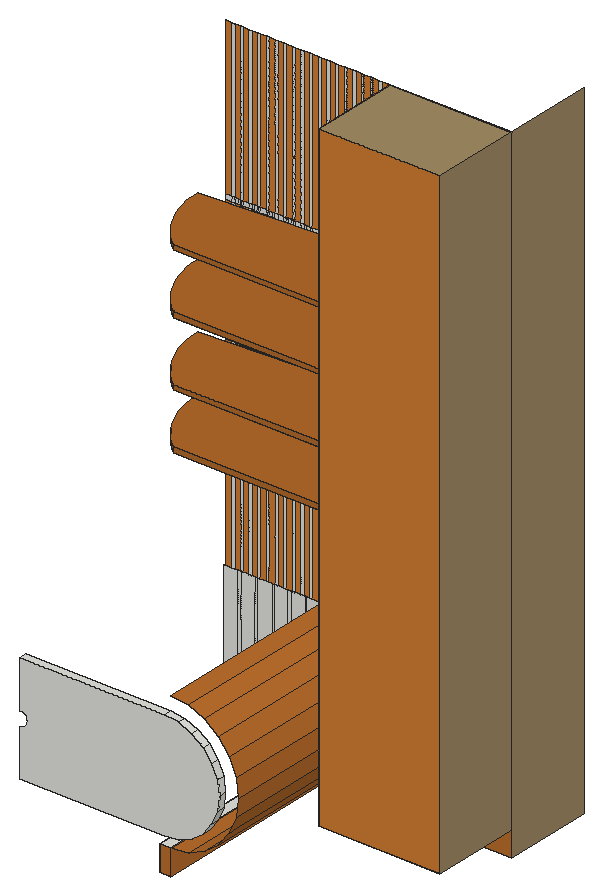
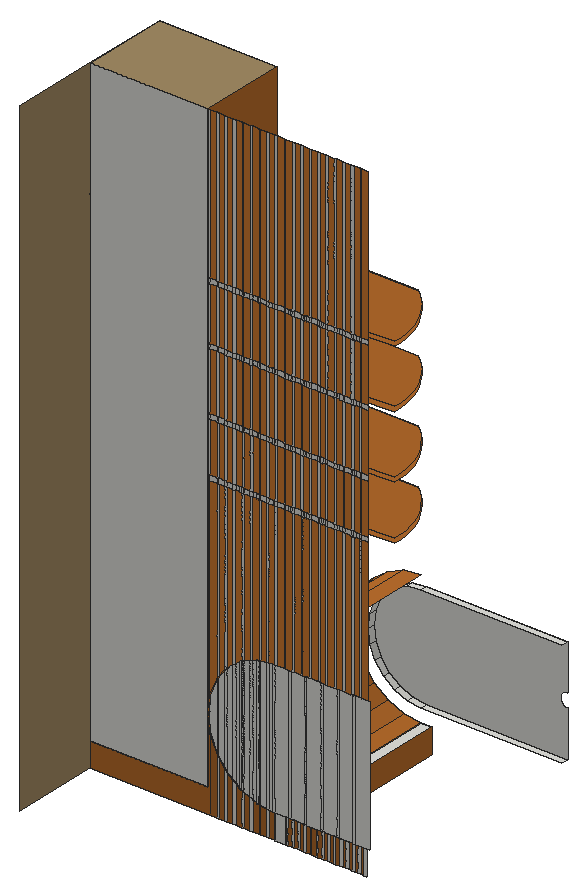
# SketchUp Ruby script. Lengths in inches.
U = 1.inch
M = Sketchup.active_model
def pt(a) = Geom::Point3d.new(a.map { |v| v * U })
def face(e, loops, mat)
  f = e.add_face(loops[0].map { |a| pt(a) })
  loops[1..].each { |l| e.add_face(l.map { |a| pt(a) }).erase! }
  f.material = f.back_material = mat if mat
  f
end
# faces: each face lists its corners as indices into pts; further lists are holes
def faces(e, pts, list, mat = nil) = list.each { |f| face(e, (f[0].is_a?(Array) ? f : [f]).map { |l| l.map { |i| pts[i] } }, mat) }
# xy, xz, yz: faces in a plane at the given z, y or x. An outline is a flat list of corners, or four numbers for a rectangle; further outlines are holes
def ring(l) = l.size == 4 ? [[l[0], l[1]], [l[2], l[1]], [l[2], l[3]], [l[0], l[3]]] : l.each_slice(2).to_a
def flat(e, list, mat, &to3) = list.each { |f| face(e, (f[0].is_a?(Array) ? f : [f]).map { |l| ring(l).map { |u, v| to3.(u, v) } }, mat) }
def xy(e, z, list, mat = nil) = flat(e, list, mat) { |x, y| [x, y, z] }
def xz(e, y, list, mat = nil) = flat(e, list, mat) { |x, z| [x, y, z] }
def yz(e, x, list, mat = nil) = flat(e, list, mat) { |y, z| [x, y, z] }
def lines(e, pts, list) = list.each { |a, b| e.add_line(pt(pts[a]), pt(pts[b])) }
# prism: a flat outline (further loops are holes) pulled along v
def prism(e, loops, v, mat = nil)
  f = face(e, loops, mat); d = Geom::Vector3d.new(v.map { |x| x * U })
  f.pushpull(f.normal.samedirection?(d) ? d.length : -d.length)
end
def box(e, o, s, mat = nil) = prism(e, [[o, [o[0] + s[0], o[1], o[2]], [o[0] + s[0], o[1] + s[1], o[2]], [o[0], o[1] + s[1], o[2]]]], [0, 0, s[2]], mat)
def at(x, y, z, deg = 0) = Geom::Transformation.translation(pt([x, y, z])) * Geom::Transformation.rotation(ORIGIN, Z_AXIS, deg.degrees)
def axes(o, x, y, z) = Geom::Transformation.new([*x, 0, *y, 0, *z, 0, *pt(o).to_a, 1])
def part(name) = M.definitions.add(name)
# library, detail: a bought-in or finely detailed component or shape, given as its bounding box
def library(name, o, s) = part(name).tap { |d| box(d.entities, o, s) }
def detail(e, o, s) = box(e.add_group.entities, o, s)
def put(e, d, t, mat = nil) = e.add_instance(d, t).tap { |i| i.material = mat if mat }
def group(e, t, mat = nil) = e.add_group.tap { |g| g.transformation = t; g.material = mat if mat }.entities
root = M.entities
M.materials.add("[Wood Bamboo]").color = [186, 110, 45]
M.materials.add("[Wood Bamboo]1").color = [211, 125, 51]
M.materials.add("[Wood Bamboo]2").color = [177, 105, 43]
M.materials.add("[Wood Floor Light]").color = [163, 140, 101]
xy(root,7.933,[[39.737,0.625,40.325,10.4375]],"[Wood Bamboo]")
xy(root,9.246,[[39.737,0.625,40.325,10.4375]])
xy(root,9.246,[[43.883,5.8125,50.1875,10.4375]],"[Wood Bamboo]")
xy(root,9.975,[[32.793,0.25,40.325,0.625]])
xy(root,15.633,[[32.793,0.25,40.325,0.625]])
xy(root,23.978,[[36.339,5.8125,36.045,6.057,35.77,6.324,35.516,6.611,35.285,6.916,35.077,7.238,34.895,7.575,34.739,7.925,34.61,8.285,34.509,8.655,34.437,9.031,34.393,9.411,34.378,9.794,34.378,10.4375,43.883,10.4375,43.883,5.8125]],"[Wood Bamboo]2")
xy(root,24.237,[[36.339,5.8125,43.883,5.8125,43.883,10.4375,34.378,10.4375,34.378,9.794,34.393,9.411,34.437,9.031,34.509,8.655,34.61,8.285,34.739,7.925,34.895,7.575,35.077,7.238,35.285,6.916,35.516,6.611,35.77,6.324,36.045,6.057]],"[Wood Bamboo]2")
xy(root,26.915,[[36.339,5.8125,36.045,6.057,35.77,6.324,35.516,6.611,35.285,6.916,35.077,7.238,34.895,7.575,34.739,7.925,34.61,8.285,34.509,8.655,34.437,9.031,34.393,9.411,34.378,9.794,34.378,10.4375,43.883,10.4375,43.883,5.8125]],"[Wood Bamboo]2")
xy(root,27.175,[[36.339,5.8125,43.883,5.8125,43.883,10.4375,34.378,10.4375,34.378,9.794,34.393,9.411,34.437,9.031,34.509,8.655,34.61,8.285,34.739,7.925,34.895,7.575,35.077,7.238,35.285,6.916,35.516,6.611,35.77,6.324,36.045,6.057]],"[Wood Bamboo]2")
xy(root,30.29,[[36.339,5.8125,36.045,6.057,35.77,6.324,35.516,6.611,35.285,6.916,35.077,7.238,34.895,7.575,34.739,7.925,34.61,8.285,34.509,8.655,34.437,9.031,34.393,9.411,34.378,9.794,34.378,10.4375,43.883,10.4375,43.883,5.8125]],"[Wood Bamboo]2")
xy(root,30.55,[[36.339,5.8125,43.883,5.8125,43.883,10.4375,34.378,10.4375,34.378,9.794,34.393,9.411,34.437,9.031,34.509,8.655,34.61,8.285,34.739,7.925,34.895,7.575,35.077,7.238,35.285,6.916,35.516,6.611,35.77,6.324,36.045,6.057]],"[Wood Bamboo]2")
xy(root,33.415,[[36.339,5.8125,36.045,6.057,35.77,6.324,35.516,6.611,35.285,6.916,35.077,7.238,34.895,7.575,34.739,7.925,34.61,8.285,34.509,8.655,34.437,9.031,34.393,9.411,34.378,9.794,34.378,10.4375,43.883,10.4375,43.883,5.8125]],"[Wood Bamboo]2")
xy(root,33.675,[[36.339,5.8125,43.883,5.8125,43.883,10.4375,34.378,10.4375,34.378,9.794,34.393,9.411,34.437,9.031,34.509,8.655,34.61,8.285,34.739,7.925,34.895,7.575,35.077,7.238,35.285,6.916,35.516,6.611,35.77,6.324,36.045,6.057]],"[Wood Bamboo]2")
xy(root,41.746,[[43.883,5.8125,50.1875,10.4375]],"[Wood Floor Light]")
xz(root,0.25,[[32.793,9.975,40.325,9.975,41.057,10.071,41.74,10.354,42.326,10.803,42.775,11.389,43.058,12.072,43.154,12.804,43.058,13.536,42.775,14.219,42.326,14.805,41.74,15.254,41.057,15.537,40.325,15.633,32.793,15.633,32.793,13.179,32.89,13.166,32.98,13.129,33.058,13.069,33.117,12.992,33.155,12.901,33.168,12.804,33.155,12.707,33.117,12.617,33.058,12.539,32.98,12.479,32.89,12.442,32.793,12.429]])
xz(root,0.625,[[39.737,7.933,40.325,9.246]],"[Wood Bamboo]")
xz(root,5.8125,[[43.883,9.246,50.1875,41.746]],"[Wood Bamboo]1")
xz(root,5.8125,[[36.339,23.978,43.883,24.237],[36.339,26.915,43.883,27.175],[36.339,30.29,43.883,30.55],[36.339,33.415,43.883,33.675]],"[Wood Bamboo]2")
xz(root,10.4375,[[35.398,7.933,35.523,9.246],[35.722,7.933,35.847,9.246],[36.046,7.933,36.171,9.246],[36.37,7.933,36.495,9.246],[36.695,7.933,36.82,9.246],
  [37.019,7.933,37.144,9.246],[37.343,7.933,37.468,9.246],[37.667,7.933,37.792,9.246],[37.991,7.933,38.116,9.246],[38.315,7.933,38.44,9.246],
  [38.639,7.933,38.764,9.246],[38.964,7.933,39.089,9.246],[39.288,7.933,39.413,9.246],[39.612,7.933,39.737,9.246],[39.737,7.933,40.303,9.246],
  [40.303,7.933,40.325,9.246],[40.605,7.933,40.73,7.933,40.73,9.299,40.605,9.283],[41.056,7.933,41.181,7.933,41.181,9.358,41.166,9.357,41.056,9.342],[41.506,7.933,41.631,7.933,41.631,9.527,41.506,9.475],[41.957,7.933,42.082,7.933,42.082,9.713,42.03,9.692,41.957,9.661],
  [42.407,7.933,42.532,7.933,42.532,10.051,42.407,9.955],[42.857,7.933,42.982,7.933,42.982,10.472,42.894,10.357,42.857,10.309],[43.308,7.933,43.433,7.933,43.433,11.088,43.407,11.025,43.308,10.896],[35.244,9.246,35.983,16.362],[35.983,9.246,36.108,16.362],
  [36.108,9.246,36.847,16.362],[36.847,9.246,36.972,16.362],[36.972,9.246,37.711,16.362],[37.711,9.246,37.836,16.362],[37.836,9.246,38.575,16.362],
  [38.575,9.246,38.7,16.362],[38.7,9.246,39.439,16.362],[39.439,9.246,39.564,16.362],[39.564,9.246,40.303,16.362],[40.303,9.246,40.325,9.246,40.428,9.259,40.428,16.349,40.325,16.362,40.303,16.362],
  [43.883,9.246,50.1875,41.746],[40.428,9.259,40.428,16.349,40.605,16.325,40.605,9.283],[40.605,9.283,40.605,16.325,40.73,16.309,40.73,9.299],[40.73,9.299,40.73,16.309,41.056,16.266,41.056,9.342],[41.056,9.342,41.056,16.266,41.166,16.251,41.166,9.357],
  [41.166,9.357,41.181,9.358,41.181,16.25,41.166,16.251],[41.181,9.358,41.246,9.367,41.291,9.386,41.291,16.222,41.246,16.241,41.181,16.25],[41.291,9.386,41.291,16.222,41.506,16.133,41.506,9.475],[41.506,9.475,41.506,16.133,41.631,16.081,41.631,9.527],[41.631,9.527,41.631,16.081,41.957,15.947,41.957,9.661],
  [41.957,9.661,41.957,15.947,42.03,15.916,42.03,9.692],[42.03,9.692,42.082,9.713,42.082,15.895,42.03,15.916],[42.082,9.713,42.104,9.723,42.155,9.762,42.155,15.846,42.104,15.886,42.082,15.895],[42.155,9.762,42.155,15.846,42.407,15.653,42.407,9.955],[42.407,9.955,42.407,15.653,42.532,15.557,42.532,10.051],
  [42.532,10.051,42.532,15.557,42.841,15.32,42.857,15.299,42.857,10.309,42.841,10.288],[42.857,10.309,42.857,15.299,42.894,15.251,42.894,10.357],[42.894,10.357,42.982,10.472,42.982,15.136,42.894,15.251],[42.982,10.472,43.019,10.52,43.019,15.088,42.982,15.136],[43.019,10.52,43.019,15.088,43.308,14.712,43.308,10.896],
  [43.308,10.896,43.308,14.712,43.407,14.583,43.433,14.52,43.433,11.088,43.407,11.025],[43.433,11.088,43.433,14.52,43.758,13.734,43.758,11.874],[43.758,11.874,43.758,13.734,43.762,13.725,43.883,12.804,43.762,11.883],[43.758,11.874,43.762,11.883,43.883,12.804,43.762,13.725,43.758,13.734],[43.883,12.804,43.883,23.978,43.758,23.978,43.758,13.734,43.762,13.725],
  [43.433,14.52,43.433,23.978,43.308,23.978,43.308,14.712,43.407,14.583],[42.982,15.136,42.982,23.978,42.857,23.978,42.857,15.299,42.894,15.251],[42.532,15.557,42.532,23.978,42.407,23.978,42.407,15.653],[42.082,15.895,42.082,23.978,41.957,23.978,41.957,15.947,42.03,15.916],[41.631,16.081,41.631,23.978,41.506,23.978,41.506,16.133],
  [41.181,16.25,41.181,23.978,41.056,23.978,41.056,16.266,41.166,16.251],[40.73,16.309,40.73,23.978,40.605,23.978,40.605,16.325],[35.65,16.362,35.775,23.978],[36.101,16.362,36.226,23.978],[36.551,16.362,36.676,23.978],
  [37.002,16.362,37.127,23.978],[37.452,16.362,37.577,23.978],[37.903,16.362,38.028,23.978],[38.353,16.362,38.478,23.978],[38.804,16.362,38.929,23.978],
  [39.254,16.362,39.379,23.978],[39.704,16.362,39.829,23.978],[40.155,16.362,40.28,23.978],[35.325,23.978,35.65,24.237],[35.65,23.978,35.775,24.237],
  [35.775,23.978,35.983,24.237],[35.983,23.978,36.101,24.237],[36.101,23.978,36.108,24.237],[36.108,23.978,36.226,24.237],[36.226,23.978,36.551,24.237],
  [36.551,23.978,36.676,24.237],[36.676,23.978,36.847,24.237],[36.847,23.978,36.972,24.237],[36.972,23.978,37.002,24.237],[37.002,23.978,37.127,24.237],
  [37.127,23.978,37.452,24.237],[37.452,23.978,37.577,24.237],[37.577,23.978,37.711,24.237],[37.711,23.978,37.836,24.237],[37.836,23.978,37.903,24.237],
  [37.903,23.978,38.028,24.237],[38.028,23.978,38.353,24.237],[38.353,23.978,38.478,24.237],[38.478,23.978,38.575,24.237],[38.575,23.978,38.7,24.237],
  [38.7,23.978,38.804,24.237],[38.804,23.978,38.929,24.237],[38.929,23.978,39.254,24.237],[39.254,23.978,39.379,24.237],[39.379,23.978,39.439,24.237],
  [39.439,23.978,39.564,24.237],[39.564,23.978,39.704,24.237],[39.704,23.978,39.829,24.237],[39.829,23.978,40.155,24.237],[40.155,23.978,40.28,24.237],
  [40.28,23.978,40.303,24.237],[40.303,23.978,40.428,24.237],[40.428,23.978,40.605,24.237],[40.605,23.978,40.73,24.237],[40.73,23.978,41.056,24.237],
  [41.056,23.978,41.166,24.237],[41.166,23.978,41.181,24.237],[41.181,23.978,41.291,24.237],[41.291,23.978,41.506,24.237],[41.506,23.978,41.631,24.237],
  [41.631,23.978,41.957,24.237],[41.957,23.978,42.03,24.237],[42.03,23.978,42.082,24.237],[42.082,23.978,42.155,24.237],[42.155,23.978,42.407,24.237],
  [42.407,23.978,42.532,24.237],[42.532,23.978,42.857,24.237],[42.857,23.978,42.894,24.237],[42.894,23.978,42.982,24.237],[42.982,23.978,43.019,24.237],
  [43.019,23.978,43.308,24.237],[43.308,23.978,43.433,24.237],[43.433,23.978,43.758,24.237],[43.758,23.978,43.883,24.237],[35.65,24.237,35.775,26.915],
  [36.101,24.237,36.226,26.915],[36.551,24.237,36.676,26.915],[37.002,24.237,37.127,26.915],[37.452,24.237,37.577,26.915],[37.903,24.237,38.028,26.915],
  [38.353,24.237,38.478,26.915],[38.804,24.237,38.929,26.915],[39.254,24.237,39.379,26.915],[39.704,24.237,39.829,26.915],[40.155,24.237,40.28,26.915],
  [40.605,24.237,40.73,26.915],[41.056,24.237,41.181,26.915],[41.506,24.237,41.631,26.915],[41.957,24.237,42.082,26.915],[42.407,24.237,42.532,26.915],
  [42.857,24.237,42.982,26.915],[43.308,24.237,43.433,26.915],[43.758,24.237,43.883,26.915],[35.325,26.915,35.65,27.175],[35.65,26.915,35.775,27.175],
  [35.775,26.915,35.983,27.175],[35.983,26.915,36.101,27.175],[36.101,26.915,36.108,27.175],[36.108,26.915,36.226,27.175],[36.226,26.915,36.551,27.175],
  [36.551,26.915,36.676,27.175],[36.676,26.915,36.847,27.175],[36.847,26.915,36.972,27.175],[36.972,26.915,37.002,27.175],[37.002,26.915,37.127,27.175],
  [37.127,26.915,37.452,27.175],[37.452,26.915,37.577,27.175],[37.577,26.915,37.711,27.175],[37.711,26.915,37.836,27.175],[37.836,26.915,37.903,27.175],
  [37.903,26.915,38.028,27.175],[38.028,26.915,38.353,27.175],[38.353,26.915,38.478,27.175],[38.478,26.915,38.575,27.175],[38.575,26.915,38.7,27.175],
  [38.7,26.915,38.804,27.175],[38.804,26.915,38.929,27.175],[38.929,26.915,39.254,27.175],[39.254,26.915,39.379,27.175],[39.379,26.915,39.439,27.175],
  [39.439,26.915,39.564,27.175],[39.564,26.915,39.704,27.175],[39.704,26.915,39.829,27.175],[39.829,26.915,40.155,27.175],[40.155,26.915,40.28,27.175],
  [40.28,26.915,40.303,27.175],[40.303,26.915,40.428,27.175],[40.428,26.915,40.605,27.175],[40.605,26.915,40.73,27.175],[40.73,26.915,41.056,27.175],
  [41.056,26.915,41.166,27.175],[41.166,26.915,41.181,27.175],[41.181,26.915,41.291,27.175],[41.291,26.915,41.506,27.175],[41.506,26.915,41.631,27.175],
  [41.631,26.915,41.957,27.175],[41.957,26.915,42.03,27.175],[42.03,26.915,42.082,27.175],[42.082,26.915,42.155,27.175],[42.155,26.915,42.407,27.175],
  [42.407,26.915,42.532,27.175],[42.532,26.915,42.857,27.175],[42.857,26.915,42.894,27.175],[42.894,26.915,42.982,27.175],[42.982,26.915,43.019,27.175],
  [43.019,26.915,43.308,27.175],[43.308,26.915,43.433,27.175],[43.433,26.915,43.758,27.175],[43.758,26.915,43.883,27.175],[35.65,27.175,35.775,30.29],
  [36.101,27.175,36.226,30.29],[36.551,27.175,36.676,30.29],[37.002,27.175,37.127,30.29],[37.452,27.175,37.577,30.29],[37.903,27.175,38.028,30.29],
  [38.353,27.175,38.478,30.29],[38.804,27.175,38.929,30.29],[39.254,27.175,39.379,30.29],[39.704,27.175,39.829,30.29],[40.155,27.175,40.28,30.29],
  [40.605,27.175,40.73,30.29],[41.056,27.175,41.181,30.29],[41.506,27.175,41.631,30.29],[41.957,27.175,42.082,30.29],[42.407,27.175,42.532,30.29],
  [42.857,27.175,42.982,30.29],[43.308,27.175,43.433,30.29],[43.758,27.175,43.883,30.29],[35.325,30.29,35.65,30.55],[35.65,30.29,35.775,30.55],
  [35.775,30.29,35.983,30.55],[35.983,30.29,36.101,30.55],[36.101,30.29,36.108,30.55],[36.108,30.29,36.226,30.55],[36.226,30.29,36.551,30.55],
  [36.551,30.29,36.676,30.55],[36.676,30.29,36.847,30.55],[36.847,30.29,36.972,30.55],[36.972,30.29,37.002,30.55],[37.002,30.29,37.127,30.55],
  [37.127,30.29,37.452,30.55],[37.452,30.29,37.577,30.55],[37.577,30.29,37.711,30.55],[37.711,30.29,37.836,30.55],[37.836,30.29,37.903,30.55],
  [37.903,30.29,38.028,30.55],[38.028,30.29,38.353,30.55],[38.353,30.29,38.478,30.55],[38.478,30.29,38.575,30.55],[38.575,30.29,38.7,30.55],
  [38.7,30.29,38.804,30.55],[38.804,30.29,38.929,30.55],[38.929,30.29,39.254,30.55],[39.254,30.29,39.379,30.55],[39.379,30.29,39.439,30.55],
  [39.439,30.29,39.564,30.55],[39.564,30.29,39.704,30.55],[39.704,30.29,39.829,30.55],[39.829,30.29,40.155,30.55],[40.155,30.29,40.28,30.55],
  [40.28,30.29,40.303,30.55],[40.303,30.29,40.428,30.55],[40.428,30.29,40.605,30.55],[40.605,30.29,40.73,30.55],[40.73,30.29,41.056,30.55],
  [41.056,30.29,41.166,30.55],[41.166,30.29,41.181,30.55],[41.181,30.29,41.291,30.55],[41.291,30.29,41.506,30.55],[41.506,30.29,41.631,30.55],
  [41.631,30.29,41.957,30.55],[41.957,30.29,42.03,30.55],[42.03,30.29,42.082,30.55],[42.082,30.29,42.155,30.55],[42.155,30.29,42.407,30.55],
  [42.407,30.29,42.532,30.55],[42.532,30.29,42.857,30.55],[42.857,30.29,42.894,30.55],[42.894,30.29,42.982,30.55],[42.982,30.29,43.019,30.55],
  [43.019,30.29,43.308,30.55],[43.308,30.29,43.433,30.55],[43.433,30.29,43.758,30.55],[43.758,30.29,43.883,30.55],[35.65,30.55,35.775,33.415],
  [36.101,30.55,36.226,33.415],[36.551,30.55,36.676,33.415],[37.002,30.55,37.127,33.415],[37.452,30.55,37.577,33.415],[37.903,30.55,38.028,33.415],
  [38.353,30.55,38.478,33.415],[38.804,30.55,38.929,33.415],[39.254,30.55,39.379,33.415],[39.704,30.55,39.829,33.415],[40.155,30.55,40.28,33.415],
  [40.605,30.55,40.73,33.415],[41.056,30.55,41.181,33.415],[41.506,30.55,41.631,33.415],[41.957,30.55,42.082,33.415],[42.407,30.55,42.532,33.415],
  [42.857,30.55,42.982,33.415],[43.308,30.55,43.433,33.415],[43.758,30.55,43.883,33.415],[35.325,33.415,35.65,33.675],[35.65,33.415,35.775,33.675],
  [35.775,33.415,35.983,33.675],[35.983,33.415,36.101,33.675],[36.101,33.415,36.108,33.675],[36.108,33.415,36.226,33.675],[36.226,33.415,36.551,33.675],
  [36.551,33.415,36.676,33.675],[36.676,33.415,36.847,33.675],[36.847,33.415,36.972,33.675],[36.972,33.415,37.002,33.675],[37.002,33.415,37.127,33.675],
  [37.127,33.415,37.452,33.675],[37.452,33.415,37.577,33.675],[37.577,33.415,37.711,33.675],[37.711,33.415,37.836,33.675],[37.836,33.415,37.903,33.675],
  [37.903,33.415,38.028,33.675],[38.028,33.415,38.353,33.675],[38.353,33.415,38.478,33.675],[38.478,33.415,38.575,33.675],[38.575,33.415,38.7,33.675],
  [38.7,33.415,38.804,33.675],[38.804,33.415,38.929,33.675],[38.929,33.415,39.254,33.675],[39.254,33.415,39.379,33.675],[39.379,33.415,39.439,33.675],
  [39.439,33.415,39.564,33.675],[39.564,33.415,39.704,33.675],[39.704,33.415,39.829,33.675],[39.829,33.415,40.155,33.675],[40.155,33.415,40.28,33.675],
  [40.28,33.415,40.303,33.675],[40.303,33.415,40.428,33.675],[40.428,33.415,40.605,33.675],[40.605,33.415,40.73,33.675],[40.73,33.415,41.056,33.675],
  [41.056,33.415,41.166,33.675],[41.166,33.415,41.181,33.675],[41.181,33.415,41.291,33.675],[41.291,33.415,41.506,33.675],[41.506,33.415,41.631,33.675],
  [41.631,33.415,41.957,33.675],[41.957,33.415,42.03,33.675],[42.03,33.415,42.082,33.675],[42.082,33.415,42.155,33.675],[42.155,33.415,42.407,33.675],
  [42.407,33.415,42.532,33.675],[42.532,33.415,42.857,33.675],[42.857,33.415,42.894,33.675],[42.894,33.415,42.982,33.675],[42.982,33.415,43.019,33.675],
  [43.019,33.415,43.308,33.675],[43.308,33.415,43.433,33.675],[43.433,33.415,43.758,33.675],[43.758,33.415,43.883,33.675],[35.65,33.675,35.775,41.746],
  [36.101,33.675,36.226,41.746],[36.551,33.675,36.676,41.746],[37.002,33.675,37.127,41.746],[37.452,33.675,37.577,41.746],[37.903,33.675,38.028,41.746],
  [38.353,33.675,38.478,41.746],[38.804,33.675,38.929,41.746],[39.254,33.675,39.379,41.746],[39.704,33.675,39.829,41.746],[40.155,33.675,40.28,41.746],
  [40.605,33.675,40.73,41.746],[41.056,33.675,41.181,41.746],[41.506,33.675,41.631,41.746],[41.957,33.675,42.082,41.746],[42.407,33.675,42.532,41.746],
  [42.857,33.675,42.982,41.746],[43.308,33.675,43.433,41.746],[43.758,33.675,43.883,41.746]])
xz(root,10.4375,[[43.758,7.933,50.1875,7.933,50.1875,9.246,43.883,9.246,43.883,12.804,43.762,11.883,43.758,11.874]],"[Wood Bamboo]")
xz(root,10.4375,[[43.758,13.734,43.758,23.978,43.433,23.978,43.433,14.52],[43.308,14.712,43.308,23.978,42.982,23.978,42.982,15.136,43.019,15.088],[42.857,15.299,42.857,23.978,42.532,23.978,42.532,15.557,42.841,15.32],[42.407,15.653,42.407,23.978,42.082,23.978,42.082,15.895,42.104,15.886,42.155,15.846],[41.957,15.947,41.957,23.978,41.631,23.978,41.631,16.081],
  [41.506,16.133,41.506,23.978,41.181,23.978,41.181,16.25,41.246,16.241,41.291,16.222],[41.056,16.266,41.056,23.978,40.73,23.978,40.73,16.309],[40.605,16.325,40.605,23.978,40.28,23.978,40.28,16.362,40.325,16.362,40.428,16.349],[35.325,16.362,35.65,23.978],[35.775,16.362,36.101,23.978],
  [36.226,16.362,36.551,23.978],[36.676,16.362,37.002,23.978],[37.127,16.362,37.452,23.978],[37.577,16.362,37.903,23.978],[38.028,16.362,38.353,23.978],
  [38.478,16.362,38.804,23.978],[38.929,16.362,39.254,23.978],[39.379,16.362,39.704,23.978],[39.829,16.362,40.155,23.978],[35.325,24.237,35.65,26.915],
  [35.775,24.237,36.101,26.915],[36.226,24.237,36.551,26.915],[36.676,24.237,37.002,26.915],[37.127,24.237,37.452,26.915],[37.577,24.237,37.903,26.915],
  [38.028,24.237,38.353,26.915],[38.478,24.237,38.804,26.915],[38.929,24.237,39.254,26.915],[39.379,24.237,39.704,26.915],[39.829,24.237,40.155,26.915],
  [40.28,24.237,40.605,26.915],[40.73,24.237,41.056,26.915],[41.181,24.237,41.506,26.915],[41.631,24.237,41.957,26.915],[42.082,24.237,42.407,26.915],
  [42.532,24.237,42.857,26.915],[42.982,24.237,43.308,26.915],[43.433,24.237,43.758,26.915],[35.325,27.175,35.65,30.29],[35.775,27.175,36.101,30.29],
  [36.226,27.175,36.551,30.29],[36.676,27.175,37.002,30.29],[37.127,27.175,37.452,30.29],[37.577,27.175,37.903,30.29],[38.028,27.175,38.353,30.29],
  [38.478,27.175,38.804,30.29],[38.929,27.175,39.254,30.29],[39.379,27.175,39.704,30.29],[39.829,27.175,40.155,30.29],[40.28,27.175,40.605,30.29],
  [40.73,27.175,41.056,30.29],[41.181,27.175,41.506,30.29],[41.631,27.175,41.957,30.29],[42.082,27.175,42.407,30.29],[42.532,27.175,42.857,30.29],
  [42.982,27.175,43.308,30.29],[43.433,27.175,43.758,30.29],[35.325,30.55,35.65,33.415],[35.775,30.55,36.101,33.415],[36.226,30.55,36.551,33.415],
  [36.676,30.55,37.002,33.415],[37.127,30.55,37.452,33.415],[37.577,30.55,37.903,33.415],[38.028,30.55,38.353,33.415],[38.478,30.55,38.804,33.415],
  [38.929,30.55,39.254,33.415],[39.379,30.55,39.704,33.415],[39.829,30.55,40.155,33.415],[40.28,30.55,40.605,33.415],[40.73,30.55,41.056,33.415],
  [41.181,30.55,41.506,33.415],[41.631,30.55,41.957,33.415],[42.082,30.55,42.407,33.415],[42.532,30.55,42.857,33.415],[42.982,30.55,43.308,33.415],
  [43.433,30.55,43.758,33.415],[35.325,33.675,35.65,41.746],[35.775,33.675,36.101,41.746],[36.226,33.675,36.551,41.746],[36.676,33.675,37.002,41.746],
  [37.127,33.675,37.452,41.746],[37.577,33.675,37.903,41.746],[38.028,33.675,38.353,41.746],[38.478,33.675,38.804,41.746],[38.929,33.675,39.254,41.746],
  [39.379,33.675,39.704,41.746],[39.829,33.675,40.155,41.746],[40.28,33.675,40.605,41.746],[40.73,33.675,41.056,41.746],[41.181,33.675,41.506,41.746],
  [41.631,33.675,41.957,41.746],[42.082,33.675,42.407,41.746],[42.532,33.675,42.857,41.746],[42.982,33.675,43.308,41.746],[43.433,33.675,43.758,41.746]],"[Wood Bamboo]1")
xz(root,10.4375,[[35.523,7.933,35.722,9.246],[35.847,7.933,36.046,9.246],[36.171,7.933,36.37,9.246],[36.495,7.933,36.695,9.246],[36.82,7.933,37.019,9.246],
  [37.144,7.933,37.343,9.246],[37.468,7.933,37.667,9.246],[37.792,7.933,37.991,9.246],[38.116,7.933,38.315,9.246],[38.44,7.933,38.639,9.246],
  [38.764,7.933,38.964,9.246],[39.089,7.933,39.288,9.246],[39.413,7.933,39.612,9.246],[40.325,7.933,40.605,7.933,40.605,9.283,40.428,9.259,40.325,9.246],[40.73,7.933,41.056,7.933,41.056,9.342,40.73,9.299],
  [41.181,7.933,41.506,7.933,41.506,9.475,41.291,9.386,41.246,9.367,41.181,9.358],[41.631,7.933,41.957,7.933,41.957,9.661,41.631,9.527],[42.082,7.933,42.407,7.933,42.407,9.955,42.155,9.762,42.104,9.723,42.082,9.713],[42.532,7.933,42.857,7.933,42.857,10.309,42.841,10.288,42.532,10.051],[42.982,7.933,43.308,7.933,43.308,10.896,43.019,10.52,42.982,10.472],
  [43.433,7.933,43.758,7.933,43.758,11.874,43.433,11.088]],"[Wood Bamboo]2")
yz(root,39.737,[[0.625,7.933,10.4375,9.246]],"[Wood Bamboo]")
yz(root,40.325,[[0.625,7.933,10.4375,9.246]],"[Wood Bamboo]")
yz(root,43.883,[[5.8125,23.978,10.4375,24.237],[5.8125,26.915,10.4375,27.175],[5.8125,30.29,10.4375,30.55],[5.8125,33.415,10.4375,33.675]])
yz(root,43.883,[[5.8125,33.675,10.4375,41.746]],"[Wood Bamboo]")
yz(root,43.883,[[5.8125,12.804,10.4375,23.978],[5.8125,24.237,10.4375,26.915],[5.8125,27.175,10.4375,30.29],[5.8125,30.55,10.4375,33.415]],"[Wood Bamboo]1")
yz(root,43.883,[[5.8125,9.246,10.4375,12.804]],"[Wood Bamboo]2")
yz(root,50.1875,[[10.4375,7.933,15.125,41.746],[5.8125,9.246,10.4375,41.746]],"[Wood Floor Light]")
p = [[40.325,10.4375,9.246],[40.428,10.4375,9.259],[40.605,10.4375,9.283],[40.73,10.4375,9.299],[41.056,10.4375,9.342],[41.166,10.4375,9.357],
  [41.181,10.4375,9.358],[41.246,10.4375,9.367],[41.246,0.625,9.367],[40.325,0.625,9.246],[41.291,10.4375,9.386],[41.506,10.4375,9.475],
  [41.631,10.4375,9.527],[41.957,10.4375,9.661],[42.03,10.4375,9.692],[42.082,10.4375,9.713],[42.104,10.4375,9.723],[42.104,0.625,9.723],
  [42.155,10.4375,9.762],[42.407,10.4375,9.955],[42.532,10.4375,10.051],[42.841,10.4375,10.288],[42.841,0.625,10.288],[40.325,0.625,9.975],
  [41.057,0.625,10.071],[41.057,0.25,10.071],[40.325,0.25,9.975],[41.74,0.625,10.354],[41.74,0.25,10.354],[42.857,10.4375,10.309],
  [42.894,10.4375,10.357],[42.982,10.4375,10.472],[43.019,10.4375,10.52],[43.308,10.4375,10.896],[43.407,10.4375,11.025],[43.407,0.625,11.025],
  [42.326,0.625,10.803],[42.326,0.25,10.803],[42.775,0.625,11.389],[42.775,0.25,11.389],[43.433,10.4375,11.088],[43.758,10.4375,11.874],
  [43.762,10.4375,11.883],[43.762,0.625,11.883],[43.058,0.625,12.072],[43.058,0.25,12.072],[43.883,10.4375,12.804],[43.883,5.8125,12.804],
  [43.883,0.625,12.804],[43.154,0.625,12.804],[43.154,0.25,12.804],[43.058,0.625,13.536],[43.058,0.25,13.536],[43.762,10.4375,13.725],
  [43.762,0.625,13.725],[42.775,0.625,14.219],[42.775,0.25,14.219],[43.758,10.4375,13.734],[43.433,10.4375,14.52],[43.407,10.4375,14.583],
  [43.407,0.625,14.583],[42.326,0.625,14.805],[42.326,0.25,14.805],[43.308,10.4375,14.712],[43.019,10.4375,15.088],[42.982,10.4375,15.136],
  [42.894,10.4375,15.251],[42.857,10.4375,15.299],[42.841,10.4375,15.32],[42.841,0.625,15.32],[41.74,0.625,15.254],[41.74,0.25,15.254],
  [41.057,0.625,15.537],[41.057,0.25,15.537],[42.532,10.4375,15.557],[42.407,10.4375,15.653],[42.155,10.4375,15.846],[42.104,10.4375,15.886],
  [42.104,0.625,15.886],[40.325,0.625,15.633],[40.325,0.25,15.633],[42.082,10.4375,15.895],[42.03,10.4375,15.916],[41.957,10.4375,15.947],
  [41.631,10.4375,16.081],[41.506,10.4375,16.133],[41.291,10.4375,16.222],[41.246,10.4375,16.241],[41.246,0.625,16.241],[41.181,10.4375,16.25],
  [41.166,10.4375,16.251],[41.056,10.4375,16.266],[40.73,10.4375,16.309],[40.605,10.4375,16.325],[40.428,10.4375,16.349],[40.325,10.4375,16.362],
  [40.325,0.625,16.362],[36.339,5.8125,24.237],[36.045,6.057,24.237],[36.045,6.057,23.978],[36.339,5.8125,23.978],[35.77,6.324,24.237],
  [35.77,6.324,23.978],[35.516,6.611,24.237],[35.516,6.611,23.978],[35.285,6.916,24.237],[35.285,6.916,23.978],[36.339,5.8125,27.175],
  [36.045,6.057,27.175],[36.045,6.057,26.915],[36.339,5.8125,26.915],[35.77,6.324,27.175],[35.77,6.324,26.915],[35.516,6.611,27.175],
  [35.516,6.611,26.915],[35.285,6.916,27.175],[35.285,6.916,26.915],[36.339,5.8125,30.55],[36.045,6.057,30.55],[36.045,6.057,30.29],
  [36.339,5.8125,30.29],[35.77,6.324,30.55],[35.77,6.324,30.29],[35.516,6.611,30.55],[35.516,6.611,30.29],[36.339,5.8125,33.675],
  [36.045,6.057,33.675],[36.045,6.057,33.415],[36.339,5.8125,33.415],[35.77,6.324,33.675],[35.77,6.324,33.415],[35.516,6.611,33.675],
  [35.516,6.611,33.415]]
faces(root,p,[[0,1,2,3,4,5,6,7,8,9],[7,10,11,12,13,14,15,16,17,8],[16,18,19,20,21,22,17],[21,29,30,31,32,33,34,35,22],[34,40,41,42,43,35],[42,46,47,48,43],[46,53,54,48,47],[53,57,58,59,60,54],
  [59,63,64,65,66,67,68,69,60],[68,74,75,76,77,78,69],[77,81,82,83,84,85,86,87,88,78],[87,89,90,91,92,93,94,95,96,88]],"[Wood Bamboo]")
faces(root,p,[[23,24,25,26],[24,27,28,25],[27,36,37,28],[36,38,39,37],[38,44,45,39],[44,49,50,45],[49,51,52,50],[51,55,56,52],
  [55,61,62,56],[61,70,71,62],[70,72,73,71],[72,79,80,73]])
faces(root,p,[[97,98,99,100],[98,101,102,99],[101,103,104,102],[103,105,106,104],[107,108,109,110],[108,111,112,109],[111,113,114,112],[113,115,116,114],
  [117,118,119,120],[118,121,122,119],[121,123,124,122],[125,126,127,128],[126,129,130,127],[129,131,132,130]],"[Wood Bamboo]2")
